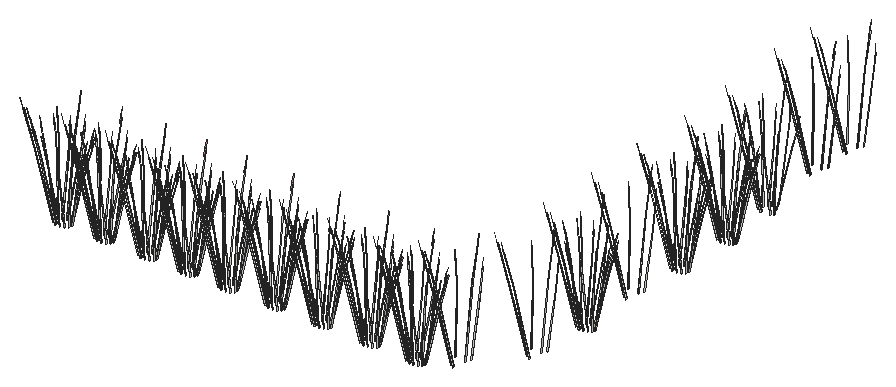
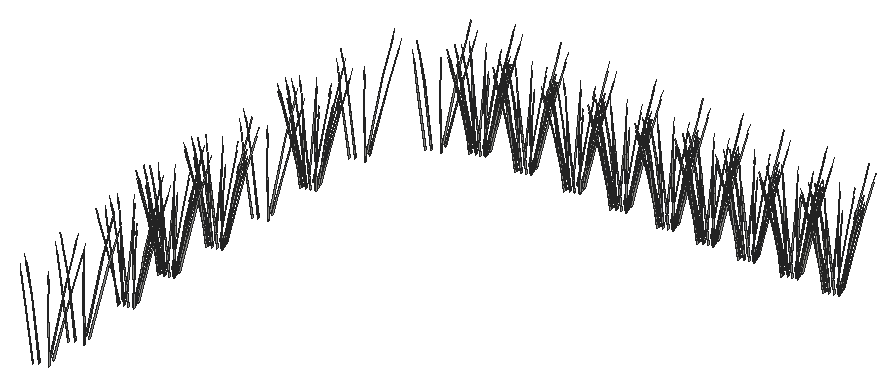
# SketchUp Ruby script. Lengths in inches.
U = 1.inch
M = Sketchup.active_model
def pt(a) = Geom::Point3d.new(a.map { |v| v * U })
def face(e, loops, mat)
  f = e.add_face(loops[0].map { |a| pt(a) })
  loops[1..].each { |l| e.add_face(l.map { |a| pt(a) }).erase! }
  f.material = f.back_material = mat if mat
  f
end
# faces: each face lists its corners as indices into pts; further lists are holes
def faces(e, pts, list, mat = nil) = list.each { |f| face(e, (f[0].is_a?(Array) ? f : [f]).map { |l| l.map { |i| pts[i] } }, mat) }
# xy, xz, yz: faces in a plane at the given z, y or x. An outline is a flat list of corners, or four numbers for a rectangle; further outlines are holes
def ring(l) = l.size == 4 ? [[l[0], l[1]], [l[2], l[1]], [l[2], l[3]], [l[0], l[3]]] : l.each_slice(2).to_a
def flat(e, list, mat, &to3) = list.each { |f| face(e, (f[0].is_a?(Array) ? f : [f]).map { |l| ring(l).map { |u, v| to3.(u, v) } }, mat) }
def xy(e, z, list, mat = nil) = flat(e, list, mat) { |x, y| [x, y, z] }
def xz(e, y, list, mat = nil) = flat(e, list, mat) { |x, z| [x, y, z] }
def yz(e, x, list, mat = nil) = flat(e, list, mat) { |y, z| [x, y, z] }
def lines(e, pts, list) = list.each { |a, b| e.add_line(pt(pts[a]), pt(pts[b])) }
# prism: a flat outline (further loops are holes) pulled along v
def prism(e, loops, v, mat = nil)
  f = face(e, loops, mat); d = Geom::Vector3d.new(v.map { |x| x * U })
  f.pushpull(f.normal.samedirection?(d) ? d.length : -d.length)
end
def box(e, o, s, mat = nil) = prism(e, [[o, [o[0] + s[0], o[1], o[2]], [o[0] + s[0], o[1] + s[1], o[2]], [o[0], o[1] + s[1], o[2]]]], [0, 0, s[2]], mat)
def at(x, y, z, deg = 0) = Geom::Transformation.translation(pt([x, y, z])) * Geom::Transformation.rotation(ORIGIN, Z_AXIS, deg.degrees)
def axes(o, x, y, z) = Geom::Transformation.new([*x, 0, *y, 0, *z, 0, *pt(o).to_a, 1])
def part(name) = M.definitions.add(name)
# library, detail: a bought-in or finely detailed component or shape, given as its bounding box
def library(name, o, s) = part(name).tap { |d| box(d.entities, o, s) }
def detail(e, o, s) = box(e.add_group.entities, o, s)
def put(e, d, t, mat = nil) = e.add_instance(d, t).tap { |i| i.material = mat if mat }
def group(e, t, mat = nil) = e.add_group.tap { |g| g.transformation = t; g.material = mat if mat }.entities
root = M.entities
M.materials.add("LightPink_Translucent").color = [144, 107, 117]
M.materials["LightPink_Translucent"].alpha = 0.75
c1 = part("blade")
p = [[2.15,0.21,22],[0,0.17,0],[0.09,0.45,0],[2.18,0.31,22],[2.29,0.31,22],[0.38,0.45,0],
  [2.48,0.24,33],[2.49,0.24,33],[2.48,0.22,33]]
faces(c1.entities,p,[[0,1,2,3],[4,5,2,3],[6,3,4,7],[8,0,3,6]])
c2 = part("seeds")
p = [[0.3,-0.1,1.38],[-0.01,-0.03,1.59],[-0.01,-0.03,0.03],[0.14,-0.07,-0.07],[0.29,-0.03,3],[0.15,0.01,3.11]]
faces(c2.entities,p,[[0,1,2,3],[1,0,4,5]],"LightPink_Translucent")
c3 = part("blade with seeds")
put(c3.entities,c1,at(0,0,0))
put(c3.entities,c2,axes([2.4,0.25,30.99],[1.5799,-0.05474,1.17369],[-0.12525,1.92788,0.29478],[-0.07173,-0.02425,1.56792]))
put(root,c3,axes([404.58,190.8125,260.05],[0.43232,0.38257,0.35414],[-0.49364,0.36215,-0.4572],[-0.25081,-0.0551,0.87481]))
put(root,c3,axes([404.87,194.07,260.05],[0.5141,-0.32171,0.35414],[0.48666,0.36734,-0.4572],[-0.07405,0.18664,0.87481]))
put(root,c3,axes([403.97,193.08,260.05],[0.66138,-0.08733,0.35414],[0.17464,0.49921,-0.4572],[-0.18953,0.13408,0.87481]))
put(root,c3,axes([407.91,194.52,260.05],[-0.11735,-0.49217,0.35414],[0.67083,-0.12996,-0.4572],[0.18018,0.14104,0.87481]))
put(root,c3,axes([409.85,191.59,260.05],[-0.66138,0.08733,0.35414],[-0.17464,-0.49921,-0.4572],[0.18953,-0.13408,0.87481]))
put(root,c3,axes([403.87,191.89,260.05],[0.63144,0.17046,0.35414],[-0.18417,0.49731,-0.4572],[-0.25423,0.0456,0.87481]))
put(root,c3,axes([408.96,190.6,260.05],[-0.5141,0.32171,0.35414],[-0.48666,-0.36734,-0.4572],[0.07405,-0.18664,0.87481]))
put(root,c3,axes([405.92,190.15,260.05],[0.11735,0.49217,0.35414],[-0.67083,0.12996,-0.4572],[-0.18018,-0.14104,0.87481]))
put(root,c3,axes([408.33,172.47,260.05],[0.22906,-0.4699,0.35414],[0.66828,0.13705,-0.4572],[0.06128,0.18919,0.87481]))
put(root,c3,axes([409.54,167.9375,260.05],[-0.22906,0.4699,0.35414],[-0.66828,-0.13705,-0.4572],[-0.06128,-0.18919,0.87481]))
put(root,c3,axes([411.27,171.73,260.05],[-0.43232,-0.38257,0.35414],[0.49364,-0.36215,-0.4572],[0.25081,0.0551,0.87481]))
put(root,c3,axes([411.98,170.66,260.05],[-0.63144,-0.17046,0.35414],[0.18417,-0.49731,-0.4572],[0.25423,-0.0456,0.87481]))
put(root,c3,axes([406.6,168.68,260.05],[0.43232,0.38257,0.35414],[-0.49364,0.36215,-0.4572],[-0.25081,-0.0551,0.87481]))
put(root,c3,axes([406.89,171.94,260.05],[0.5141,-0.32171,0.35414],[0.48666,0.36734,-0.4572],[-0.07405,0.18664,0.87481]))
put(root,c3,axes([405.99,170.95,260.05],[0.66138,-0.08733,0.35414],[0.17464,0.49921,-0.4572],[-0.18953,0.13408,0.87481]))
put(root,c3,axes([409.93,172.39,260.05],[-0.11735,-0.49217,0.35414],[0.67083,-0.12996,-0.4572],[0.18018,0.14104,0.87481]))
put(root,c3,axes([411.875,169.46,260.05],[-0.66138,0.08733,0.35414],[-0.17464,-0.49921,-0.4572],[0.18953,-0.13408,0.87481]))
put(root,c3,axes([405.89,169.75,260.05],[0.63144,0.17046,0.35414],[-0.18417,0.49731,-0.4572],[-0.25423,0.0456,0.87481]))
put(root,c3,axes([410.98,168.47,260.05],[-0.5141,0.32171,0.35414],[-0.48666,-0.36734,-0.4572],[0.07405,-0.18664,0.87481]))
put(root,c3,axes([407.93,168.02,260.05],[0.11735,0.49217,0.35414],[-0.67083,0.12996,-0.4572],[-0.18018,-0.14104,0.87481]))
put(root,c3,axes([407.96,149.88,260.05],[0.22906,-0.4699,0.35414],[0.66828,0.13705,-0.4572],[0.06128,0.18919,0.87481]))
put(root,c3,axes([409.18,145.35,260.05],[-0.22906,0.4699,0.35414],[-0.66828,-0.13705,-0.4572],[-0.06128,-0.18919,0.87481]))
put(root,c3,axes([410.91,149.14,260.05],[-0.43232,-0.38257,0.35414],[0.49364,-0.36215,-0.4572],[0.25081,0.0551,0.87481]))
put(root,c3,axes([411.62,148.0625,260.05],[-0.63144,-0.17046,0.35414],[0.18417,-0.49731,-0.4572],[0.25423,-0.0456,0.87481]))
put(root,c3,axes([406.24,146.09,260.05],[0.43232,0.38257,0.35414],[-0.49364,0.36215,-0.4572],[-0.25081,-0.0551,0.87481]))
put(root,c3,axes([406.52,149.35,260.05],[0.5141,-0.32171,0.35414],[0.48666,0.36734,-0.4572],[-0.07405,0.18664,0.87481]))
put(root,c3,axes([405.63,148.35,260.05],[0.66138,-0.08733,0.35414],[0.17464,0.49921,-0.4572],[-0.18953,0.13408,0.87481]))
put(root,c3,axes([409.57,149.8,260.05],[-0.11735,-0.49217,0.35414],[0.67083,-0.12996,-0.4572],[0.18018,0.14104,0.87481]))
put(root,c3,axes([411.51,146.87,260.05],[-0.66138,0.08733,0.35414],[-0.17464,-0.49921,-0.4572],[0.18953,-0.13408,0.87481]))
put(root,c3,axes([405.52,147.16,260.05],[0.63144,0.17046,0.35414],[-0.18417,0.49731,-0.4572],[-0.25423,0.0456,0.87481]))
put(root,c3,axes([410.62,145.875,260.05],[-0.5141,0.32171,0.35414],[-0.48666,-0.36734,-0.4572],[0.07405,-0.18664,0.87481]))
put(root,c3,axes([407.57,145.42,260.05],[0.11735,0.49217,0.35414],[-0.67083,0.12996,-0.4572],[-0.18018,-0.14104,0.87481]))
put(root,c3,axes([408.46,104.08,260.05],[0.22906,-0.4699,0.35414],[0.66828,0.13705,-0.4572],[0.06128,0.18919,0.87481]))
put(root,c3,axes([409.67,99.55,260.05],[-0.22906,0.4699,0.35414],[-0.66828,-0.13705,-0.4572],[-0.06128,-0.18919,0.87481]))
put(root,c3,axes([411.4,103.34,260.05],[-0.43232,-0.38257,0.35414],[0.49364,-0.36215,-0.4572],[0.25081,0.0551,0.87481]))
put(root,c3,axes([412.11,102.27,260.05],[-0.63144,-0.17046,0.35414],[0.18417,-0.49731,-0.4572],[0.25423,-0.0456,0.87481]))
put(root,c3,axes([406.73,100.29,260.05],[0.43232,0.38257,0.35414],[-0.49364,0.36215,-0.4572],[-0.25081,-0.0551,0.87481]))
put(root,c3,axes([407.02,103.55,260.05],[0.5141,-0.32171,0.35414],[0.48666,0.36734,-0.4572],[-0.07405,0.18664,0.87481]))
put(root,c3,axes([406.125,102.56,260.05],[0.66138,-0.08733,0.35414],[0.17464,0.49921,-0.4572],[-0.18953,0.13408,0.87481]))
put(root,c3,axes([410.07,104,260.05],[-0.11735,-0.49217,0.35414],[0.67083,-0.12996,-0.4572],[0.18018,0.14104,0.87481]))
put(root,c3,axes([412.01,101.07,260.05],[-0.66138,0.08733,0.35414],[-0.17464,-0.49921,-0.4572],[0.18953,-0.13408,0.87481]))
put(root,c3,axes([406.02,101.36,260.05],[0.63144,0.17046,0.35414],[-0.18417,0.49731,-0.4572],[-0.25423,0.0456,0.87481]))
put(root,c3,axes([411.12,100.08,260.05],[-0.5141,0.32171,0.35414],[-0.48666,-0.36734,-0.4572],[0.07405,-0.18664,0.87481]))
put(root,c3,axes([408.07,99.625,260.05],[0.11735,0.49217,0.35414],[-0.67083,0.12996,-0.4572],[-0.18018,-0.14104,0.87481]))
put(root,c3,axes([381.59,55.89,260.05],[0.22906,-0.4699,0.35414],[0.66828,0.13705,-0.4572],[0.06128,0.18919,0.87481]))
put(root,c3,axes([382.8,51.36,260.05],[-0.22906,0.4699,0.35414],[-0.66828,-0.13705,-0.4572],[-0.06128,-0.18919,0.87481]))
put(root,c3,axes([384.53,55.15,260.05],[-0.43232,-0.38257,0.35414],[0.49364,-0.36215,-0.4572],[0.25081,0.0551,0.87481]))
put(root,c3,axes([385.24,54.08,260.05],[-0.63144,-0.17046,0.35414],[0.18417,-0.49731,-0.4572],[0.25423,-0.0456,0.87481]))
put(root,c3,axes([379.86,52.1,260.05],[0.43232,0.38257,0.35414],[-0.49364,0.36215,-0.4572],[-0.25081,-0.0551,0.87481]))
put(root,c3,axes([380.15,55.37,260.05],[0.5141,-0.32171,0.35414],[0.48666,0.36734,-0.4572],[-0.07405,0.18664,0.87481]))
put(root,c3,axes([379.25,54.37,260.05],[0.66138,-0.08733,0.35414],[0.17464,0.49921,-0.4572],[-0.18953,0.13408,0.87481]))
put(root,c3,axes([383.19,55.82,260.05],[-0.11735,-0.49217,0.35414],[0.67083,-0.12996,-0.4572],[0.18018,0.14104,0.87481]))
put(root,c3,axes([385.14,52.89,260.05],[-0.66138,0.08733,0.35414],[-0.17464,-0.49921,-0.4572],[0.18953,-0.13408,0.87481]))
put(root,c3,axes([379.15,53.18,260.05],[0.63144,0.17046,0.35414],[-0.18417,0.49731,-0.4572],[-0.25423,0.0456,0.87481]))
put(root,c3,axes([384.24,51.89,260.05],[-0.5141,0.32171,0.35414],[-0.48666,-0.36734,-0.4572],[0.07405,-0.18664,0.87481]))
put(root,c3,axes([381.2,51.4375,260.05],[0.11735,0.49217,0.35414],[-0.67083,0.12996,-0.4572],[-0.18018,-0.14104,0.87481]))
put(root,c3,axes([363.95,55.89,260.05],[0.22906,-0.4699,0.35414],[0.66828,0.13705,-0.4572],[0.06128,0.18919,0.87481]))
put(root,c3,axes([365.16,51.36,260.05],[-0.22906,0.4699,0.35414],[-0.66828,-0.13705,-0.4572],[-0.06128,-0.18919,0.87481]))
put(root,c3,axes([366.89,55.15,260.05],[-0.43232,-0.38257,0.35414],[0.49364,-0.36215,-0.4572],[0.25081,0.0551,0.87481]))
put(root,c3,axes([367.6,54.08,260.05],[-0.63144,-0.17046,0.35414],[0.18417,-0.49731,-0.4572],[0.25423,-0.0456,0.87481]))
put(root,c3,axes([362.22,52.1,260.05],[0.43232,0.38257,0.35414],[-0.49364,0.36215,-0.4572],[-0.25081,-0.0551,0.87481]))
put(root,c3,axes([362.51,55.37,260.05],[0.5141,-0.32171,0.35414],[0.48666,0.36734,-0.4572],[-0.07405,0.18664,0.87481]))
put(root,c3,axes([361.62,54.37,260.05],[0.66138,-0.08733,0.35414],[0.17464,0.49921,-0.4572],[-0.18953,0.13408,0.87481]))
put(root,c3,axes([365.56,55.82,260.05],[-0.11735,-0.49217,0.35414],[0.67083,-0.12996,-0.4572],[0.18018,0.14104,0.87481]))
put(root,c3,axes([367.5,52.89,260.05],[-0.66138,0.08733,0.35414],[-0.17464,-0.49921,-0.4572],[0.18953,-0.13408,0.87481]))
put(root,c3,axes([361.51,53.18,260.05],[0.63144,0.17046,0.35414],[-0.18417,0.49731,-0.4572],[-0.25423,0.0456,0.87481]))
put(root,c3,axes([366.61,51.89,260.05],[-0.5141,0.32171,0.35414],[-0.48666,-0.36734,-0.4572],[0.07405,-0.18664,0.87481]))
put(root,c3,axes([363.5625,51.4375,260.05],[0.11735,0.49217,0.35414],[-0.67083,0.12996,-0.4572],[-0.18018,-0.14104,0.87481]))
put(root,c3,axes([345.17,55.89,260.05],[0.22906,-0.4699,0.35414],[0.66828,0.13705,-0.4572],[0.06128,0.18919,0.87481]))
put(root,c3,axes([346.38,51.36,260.05],[-0.22906,0.4699,0.35414],[-0.66828,-0.13705,-0.4572],[-0.06128,-0.18919,0.87481]))
put(root,c3,axes([348.11,55.15,260.05],[-0.43232,-0.38257,0.35414],[0.49364,-0.36215,-0.4572],[0.25081,0.0551,0.87481]))
put(root,c3,axes([348.82,54.08,260.05],[-0.63144,-0.17046,0.35414],[0.18417,-0.49731,-0.4572],[0.25423,-0.0456,0.87481]))
put(root,c3,axes([343.44,52.1,260.05],[0.43232,0.38257,0.35414],[-0.49364,0.36215,-0.4572],[-0.25081,-0.0551,0.87481]))
put(root,c3,axes([343.73,55.37,260.05],[0.5141,-0.32171,0.35414],[0.48666,0.36734,-0.4572],[-0.07405,0.18664,0.87481]))
put(root,c3,axes([342.84,54.37,260.05],[0.66138,-0.08733,0.35414],[0.17464,0.49921,-0.4572],[-0.18953,0.13408,0.87481]))
put(root,c3,axes([346.77,55.82,260.05],[-0.11735,-0.49217,0.35414],[0.67083,-0.12996,-0.4572],[0.18018,0.14104,0.87481]))
put(root,c3,axes([348.72,52.89,260.05],[-0.66138,0.08733,0.35414],[-0.17464,-0.49921,-0.4572],[0.18953,-0.13408,0.87481]))
put(root,c3,axes([342.73,53.18,260.05],[0.63144,0.17046,0.35414],[-0.18417,0.49731,-0.4572],[-0.25423,0.0456,0.87481]))
put(root,c3,axes([347.82,51.89,260.05],[-0.5141,0.32171,0.35414],[-0.48666,-0.36734,-0.4572],[0.07405,-0.18664,0.87481]))
put(root,c3,axes([344.78,51.4375,260.05],[0.11735,0.49217,0.35414],[-0.67083,0.12996,-0.4572],[-0.18018,-0.14104,0.87481]))
put(root,c3,axes([327.26,55.89,260.05],[0.22906,-0.4699,0.35414],[0.66828,0.13705,-0.4572],[0.06128,0.18919,0.87481]))
put(root,c3,axes([328.48,51.36,260.05],[-0.22906,0.4699,0.35414],[-0.66828,-0.13705,-0.4572],[-0.06128,-0.18919,0.87481]))
put(root,c3,axes([330.2,55.15,260.05],[-0.43232,-0.38257,0.35414],[0.49364,-0.36215,-0.4572],[0.25081,0.0551,0.87481]))
put(root,c3,axes([330.92,54.08,260.05],[-0.63144,-0.17046,0.35414],[0.18417,-0.49731,-0.4572],[0.25423,-0.0456,0.87481]))
put(root,c3,axes([325.54,52.1,260.05],[0.43232,0.38257,0.35414],[-0.49364,0.36215,-0.4572],[-0.25081,-0.0551,0.87481]))
put(root,c3,axes([325.82,55.37,260.05],[0.5141,-0.32171,0.35414],[0.48666,0.36734,-0.4572],[-0.07405,0.18664,0.87481]))
put(root,c3,axes([324.93,54.37,260.05],[0.66138,-0.08733,0.35414],[0.17464,0.49921,-0.4572],[-0.18953,0.13408,0.87481]))
put(root,c3,axes([328.87,55.82,260.05],[-0.11735,-0.49217,0.35414],[0.67083,-0.12996,-0.4572],[0.18018,0.14104,0.87481]))
put(root,c3,axes([330.8125,52.89,260.05],[-0.66138,0.08733,0.35414],[-0.17464,-0.49921,-0.4572],[0.18953,-0.13408,0.87481]))
put(root,c3,axes([324.82,53.18,260.05],[0.63144,0.17046,0.35414],[-0.18417,0.49731,-0.4572],[-0.25423,0.0456,0.87481]))
put(root,c3,axes([329.92,51.89,260.05],[-0.5141,0.32171,0.35414],[-0.48666,-0.36734,-0.4572],[0.07405,-0.18664,0.87481]))
put(root,c3,axes([326.87,51.4375,260.05],[0.11735,0.49217,0.35414],[-0.67083,0.12996,-0.4572],[-0.18018,-0.14104,0.87481]))
put(root,c3,axes([309.16,55.89,260.05],[0.22906,-0.4699,0.35414],[0.66828,0.13705,-0.4572],[0.06128,0.18919,0.87481]))
put(root,c3,axes([310.37,51.36,260.05],[-0.22906,0.4699,0.35414],[-0.66828,-0.13705,-0.4572],[-0.06128,-0.18919,0.87481]))
put(root,c3,axes([312.1,55.15,260.05],[-0.43232,-0.38257,0.35414],[0.49364,-0.36215,-0.4572],[0.25081,0.0551,0.87481]))
put(root,c3,axes([312.81,54.08,260.05],[-0.63144,-0.17046,0.35414],[0.18417,-0.49731,-0.4572],[0.25423,-0.0456,0.87481]))
put(root,c3,axes([307.43,52.1,260.05],[0.43232,0.38257,0.35414],[-0.49364,0.36215,-0.4572],[-0.25081,-0.0551,0.87481]))
put(root,c3,axes([307.71,55.37,260.05],[0.5141,-0.32171,0.35414],[0.48666,0.36734,-0.4572],[-0.07405,0.18664,0.87481]))
put(root,c3,axes([306.82,54.37,260.05],[0.66138,-0.08733,0.35414],[0.17464,0.49921,-0.4572],[-0.18953,0.13408,0.87481]))
put(root,c3,axes([310.76,55.82,260.05],[-0.11735,-0.49217,0.35414],[0.67083,-0.12996,-0.4572],[0.18018,0.14104,0.87481]))
put(root,c3,axes([312.7,52.89,260.05],[-0.66138,0.08733,0.35414],[-0.17464,-0.49921,-0.4572],[0.18953,-0.13408,0.87481]))
put(root,c3,axes([306.72,53.18,260.05],[0.63144,0.17046,0.35414],[-0.18417,0.49731,-0.4572],[-0.25423,0.0456,0.87481]))
put(root,c3,axes([311.81,51.89,260.05],[-0.5141,0.32171,0.35414],[-0.48666,-0.36734,-0.4572],[0.07405,-0.18664,0.87481]))
put(root,c3,axes([308.76,51.4375,260.05],[0.11735,0.49217,0.35414],[-0.67083,0.12996,-0.4572],[-0.18018,-0.14104,0.87481]))
put(root,c3,axes([293.71,55.89,260.05],[0.22906,-0.4699,0.35414],[0.66828,0.13705,-0.4572],[0.06128,0.18919,0.87481]))
put(root,c3,axes([294.92,51.36,260.05],[-0.22906,0.4699,0.35414],[-0.66828,-0.13705,-0.4572],[-0.06128,-0.18919,0.87481]))
put(root,c3,axes([296.65,55.15,260.05],[-0.43232,-0.38257,0.35414],[0.49364,-0.36215,-0.4572],[0.25081,0.0551,0.87481]))
put(root,c3,axes([297.36,54.08,260.05],[-0.63144,-0.17046,0.35414],[0.18417,-0.49731,-0.4572],[0.25423,-0.0456,0.87481]))
put(root,c3,axes([291.98,52.1,260.05],[0.43232,0.38257,0.35414],[-0.49364,0.36215,-0.4572],[-0.25081,-0.0551,0.87481]))
put(root,c3,axes([292.27,55.37,260.05],[0.5141,-0.32171,0.35414],[0.48666,0.36734,-0.4572],[-0.07405,0.18664,0.87481]))
put(root,c3,axes([291.375,54.37,260.05],[0.66138,-0.08733,0.35414],[0.17464,0.49921,-0.4572],[-0.18953,0.13408,0.87481]))
put(root,c3,axes([295.3125,55.82,260.05],[-0.11735,-0.49217,0.35414],[0.67083,-0.12996,-0.4572],[0.18018,0.14104,0.87481]))
put(root,c3,axes([297.25,52.89,260.05],[-0.66138,0.08733,0.35414],[-0.17464,-0.49921,-0.4572],[0.18953,-0.13408,0.87481]))
put(root,c3,axes([291.27,53.18,260.05],[0.63144,0.17046,0.35414],[-0.18417,0.49731,-0.4572],[-0.25423,0.0456,0.87481]))
put(root,c3,axes([296.36,51.89,260.05],[-0.5141,0.32171,0.35414],[-0.48666,-0.36734,-0.4572],[0.07405,-0.18664,0.87481]))
put(root,c3,axes([293.32,51.4375,260.05],[0.11735,0.49217,0.35414],[-0.67083,0.12996,-0.4572],[-0.18018,-0.14104,0.87481]))
put(root,c3,axes([277.98,55.89,260.05],[0.22906,-0.4699,0.35414],[0.66828,0.13705,-0.4572],[0.06128,0.18919,0.87481]))
put(root,c3,axes([279.19,51.36,260.05],[-0.22906,0.4699,0.35414],[-0.66828,-0.13705,-0.4572],[-0.06128,-0.18919,0.87481]))
put(root,c3,axes([280.92,55.15,260.05],[-0.43232,-0.38257,0.35414],[0.49364,-0.36215,-0.4572],[0.25081,0.0551,0.87481]))
put(root,c3,axes([281.63,54.08,260.05],[-0.63144,-0.17046,0.35414],[0.18417,-0.49731,-0.4572],[0.25423,-0.0456,0.87481]))
put(root,c3,axes([276.25,52.1,260.05],[0.43232,0.38257,0.35414],[-0.49364,0.36215,-0.4572],[-0.25081,-0.0551,0.87481]))
put(root,c3,axes([276.54,55.37,260.05],[0.5141,-0.32171,0.35414],[0.48666,0.36734,-0.4572],[-0.07405,0.18664,0.87481]))
put(root,c3,axes([275.65,54.37,260.05],[0.66138,-0.08733,0.35414],[0.17464,0.49921,-0.4572],[-0.18953,0.13408,0.87481]))
put(root,c3,axes([279.58,55.82,260.05],[-0.11735,-0.49217,0.35414],[0.67083,-0.12996,-0.4572],[0.18018,0.14104,0.87481]))
put(root,c3,axes([281.53,52.89,260.05],[-0.66138,0.08733,0.35414],[-0.17464,-0.49921,-0.4572],[0.18953,-0.13408,0.87481]))
put(root,c3,axes([275.54,53.18,260.05],[0.63144,0.17046,0.35414],[-0.18417,0.49731,-0.4572],[-0.25423,0.0456,0.87481]))
put(root,c3,axes([280.63,51.89,260.05],[-0.5141,0.32171,0.35414],[-0.48666,-0.36734,-0.4572],[0.07405,-0.18664,0.87481]))
put(root,c3,axes([277.59,51.4375,260.05],[0.11735,0.49217,0.35414],[-0.67083,0.12996,-0.4572],[-0.18018,-0.14104,0.87481]))
put(root,c3,axes([261.25,55.89,260.05],[0.22906,-0.4699,0.35414],[0.66828,0.13705,-0.4572],[0.06128,0.18919,0.87481]))
put(root,c3,axes([262.46,51.36,260.05],[-0.22906,0.4699,0.35414],[-0.66828,-0.13705,-0.4572],[-0.06128,-0.18919,0.87481]))
put(root,c3,axes([264.19,55.15,260.05],[-0.43232,-0.38257,0.35414],[0.49364,-0.36215,-0.4572],[0.25081,0.0551,0.87481]))
put(root,c3,axes([264.9,54.08,260.05],[-0.63144,-0.17046,0.35414],[0.18417,-0.49731,-0.4572],[0.25423,-0.0456,0.87481]))
put(root,c3,axes([259.52,52.1,260.05],[0.43232,0.38257,0.35414],[-0.49364,0.36215,-0.4572],[-0.25081,-0.0551,0.87481]))
put(root,c3,axes([259.81,55.37,260.05],[0.5141,-0.32171,0.35414],[0.48666,0.36734,-0.4572],[-0.07405,0.18664,0.87481]))
put(root,c3,axes([258.92,54.37,260.05],[0.66138,-0.08733,0.35414],[0.17464,0.49921,-0.4572],[-0.18953,0.13408,0.87481]))
put(root,c3,axes([262.86,55.82,260.05],[-0.11735,-0.49217,0.35414],[0.67083,-0.12996,-0.4572],[0.18018,0.14104,0.87481]))
put(root,c3,axes([264.8,52.89,260.05],[-0.66138,0.08733,0.35414],[-0.17464,-0.49921,-0.4572],[0.18953,-0.13408,0.87481]))
put(root,c3,axes([258.8125,53.18,260.05],[0.63144,0.17046,0.35414],[-0.18417,0.49731,-0.4572],[-0.25423,0.0456,0.87481]))
put(root,c3,axes([263.91,51.89,260.05],[-0.5141,0.32171,0.35414],[-0.48666,-0.36734,-0.4572],[0.07405,-0.18664,0.87481]))
put(root,c3,axes([260.86,51.4375,260.05],[0.11735,0.49217,0.35414],[-0.67083,0.12996,-0.4572],[-0.18018,-0.14104,0.87481]))
put(root,c3,axes([245.1875,55.89,260.05],[0.22906,-0.4699,0.35414],[0.66828,0.13705,-0.4572],[0.06128,0.18919,0.87481]))
put(root,c3,axes([246.4,51.36,260.05],[-0.22906,0.4699,0.35414],[-0.66828,-0.13705,-0.4572],[-0.06128,-0.18919,0.87481]))
put(root,c3,axes([248.13,55.15,260.05],[-0.43232,-0.38257,0.35414],[0.49364,-0.36215,-0.4572],[0.25081,0.0551,0.87481]))
put(root,c3,axes([248.84,54.08,260.05],[-0.63144,-0.17046,0.35414],[0.18417,-0.49731,-0.4572],[0.25423,-0.0456,0.87481]))
put(root,c3,axes([243.46,52.1,260.05],[0.43232,0.38257,0.35414],[-0.49364,0.36215,-0.4572],[-0.25081,-0.0551,0.87481]))
put(root,c3,axes([243.74,55.37,260.05],[0.5141,-0.32171,0.35414],[0.48666,0.36734,-0.4572],[-0.07405,0.18664,0.87481]))
put(root,c3,axes([242.85,54.37,260.05],[0.66138,-0.08733,0.35414],[0.17464,0.49921,-0.4572],[-0.18953,0.13408,0.87481]))
put(root,c3,axes([246.79,55.82,260.05],[-0.11735,-0.49217,0.35414],[0.67083,-0.12996,-0.4572],[0.18018,0.14104,0.87481]))
put(root,c3,axes([248.73,52.89,260.05],[-0.66138,0.08733,0.35414],[-0.17464,-0.49921,-0.4572],[0.18953,-0.13408,0.87481]))
put(root,c3,axes([242.75,53.18,260.05],[0.63144,0.17046,0.35414],[-0.18417,0.49731,-0.4572],[-0.25423,0.0456,0.87481]))
put(root,c3,axes([247.84,51.89,260.05],[-0.5141,0.32171,0.35414],[-0.48666,-0.36734,-0.4572],[0.07405,-0.18664,0.87481]))
put(root,c3,axes([244.79,51.4375,260.05],[0.11735,0.49217,0.35414],[-0.67083,0.12996,-0.4572],[-0.18018,-0.14104,0.87481]))
put(root,c3,axes([403.9,221.74,260.0625],[-0.74868,-0.15974,0.53283],[0.25601,-0.52518,0.43934],[0.04499,0.20653,1.10256]))
put(root,c3,axes([408.23,127.85,260.0625],[-0.74868,-0.15974,0.53283],[0.25601,-0.52518,0.43934],[0.04499,0.20653,1.10256]))
put(root,c3,axes([408.33,80.94,260.0625],[-0.74868,-0.15974,0.53283],[0.25601,-0.52518,0.43934],[0.04499,0.20653,1.10256]))
put(root,c3,axes([393.71,62.51,260.0625],[-0.74868,-0.15974,0.53283],[0.25601,-0.52518,0.43934],[0.04499,0.20653,1.10256]))
put(root,c3,axes([404.05,238.8125,260.0625],[-0.74868,-0.15974,0.53283],[0.25601,-0.52518,0.43934],[0.04499,0.20653,1.10256]))
put(root,c3,axes([406.3,194.99,260.0625],[-0.74868,-0.15974,0.53283],[0.25601,-0.52518,0.43934],[0.04499,0.20653,1.10256]))
put(root,c3,axes([408.32,172.86,260.0625],[-0.74868,-0.15974,0.53283],[0.25601,-0.52518,0.43934],[0.04499,0.20653,1.10256]))
put(root,c3,axes([407.96,150.26,260.0625],[-0.74868,-0.15974,0.53283],[0.25601,-0.52518,0.43934],[0.04499,0.20653,1.10256]))
put(root,c3,axes([408.45,104.47,260.0625],[-0.74868,-0.15974,0.53283],[0.25601,-0.52518,0.43934],[0.04499,0.20653,1.10256]))
put(root,c3,axes([381.58,56.28,260.0625],[-0.74868,-0.15974,0.53283],[0.25601,-0.52518,0.43934],[0.04499,0.20653,1.10256]))
put(root,c3,axes([363.94,56.28,260.0625],[-0.74868,-0.15974,0.53283],[0.25601,-0.52518,0.43934],[0.04499,0.20653,1.10256]))
put(root,c3,axes([345.16,56.28,260.0625],[-0.74868,-0.15974,0.53283],[0.25601,-0.52518,0.43934],[0.04499,0.20653,1.10256]))
put(root,c3,axes([327.25,56.28,260.0625],[-0.74868,-0.15974,0.53283],[0.25601,-0.52518,0.43934],[0.04499,0.20653,1.10256]))
put(root,c3,axes([309.15,56.28,260.0625],[-0.74868,-0.15974,0.53283],[0.25601,-0.52518,0.43934],[0.04499,0.20653,1.10256]))
put(root,c3,axes([293.7,56.28,260.0625],[-0.74868,-0.15974,0.53283],[0.25601,-0.52518,0.43934],[0.04499,0.20653,1.10256]))
put(root,c3,axes([277.97,56.28,260.0625],[-0.74868,-0.15974,0.53283],[0.25601,-0.52518,0.43934],[0.04499,0.20653,1.10256]))
put(root,c3,axes([261.24,56.28,260.0625],[-0.74868,-0.15974,0.53283],[0.25601,-0.52518,0.43934],[0.04499,0.20653,1.10256]))
put(root,c3,axes([245.18,56.28,260.0625],[-0.74868,-0.15974,0.53283],[0.25601,-0.52518,0.43934],[0.04499,0.20653,1.10256]))
put(root,c3,axes([401.5,217.22,260.09],[0.62747,-0.45094,0.53763],[0.54116,0.47889,0.4433],[-0.29439,-0.08318,1.11249]))
put(root,c3,axes([403.21,216.32,260.09],[0.84639,-0.15705,0.53763],[0.14689,0.61608,0.4433],[-0.19906,-0.18157,1.11249]))
put(root,c3,axes([405.84,123.33,260.09],[0.62747,-0.45094,0.53763],[0.54116,0.47889,0.4433],[-0.29439,-0.08318,1.11249]))
put(root,c3,axes([407.55,122.43,260.09],[0.84639,-0.15705,0.53763],[0.14689,0.61608,0.4433],[-0.19906,-0.18157,1.11249]))
put(root,c3,axes([405.93,76.42,260.09],[0.62747,-0.45094,0.53763],[0.54116,0.47889,0.4433],[-0.29439,-0.08318,1.11249]))
put(root,c3,axes([407.64,75.52,260.09],[0.84639,-0.15705,0.53763],[0.14689,0.61608,0.4433],[-0.19906,-0.18157,1.11249]))
put(root,c3,axes([391.3125,57.99,260.09],[0.62747,-0.45094,0.53763],[0.54116,0.47889,0.4433],[-0.29439,-0.08318,1.11249]))
put(root,c3,axes([393.03,57.09,260.09],[0.84639,-0.15705,0.53763],[0.14689,0.61608,0.4433],[-0.19906,-0.18157,1.11249]))
put(root,c3,axes([401.66,234.29,260.09],[0.62747,-0.45094,0.53763],[0.54116,0.47889,0.4433],[-0.29439,-0.08318,1.11249]))
put(root,c3,axes([403.37,233.39,260.09],[0.84639,-0.15705,0.53763],[0.14689,0.61608,0.4433],[-0.19906,-0.18157,1.11249]))
put(root,c3,axes([403.9,190.47,260.09],[0.62747,-0.45094,0.53763],[0.54116,0.47889,0.4433],[-0.29439,-0.08318,1.11249]))
put(root,c3,axes([405.61,189.57,260.09],[0.84639,-0.15705,0.53763],[0.14689,0.61608,0.4433],[-0.19906,-0.18157,1.11249]))
put(root,c3,axes([405.92,168.34,260.09],[0.62747,-0.45094,0.53763],[0.54116,0.47889,0.4433],[-0.29439,-0.08318,1.11249]))
put(root,c3,axes([407.63,167.4375,260.09],[0.84639,-0.15705,0.53763],[0.14689,0.61608,0.4433],[-0.19906,-0.18157,1.11249]))
put(root,c3,axes([405.56,145.74,260.09],[0.62747,-0.45094,0.53763],[0.54116,0.47889,0.4433],[-0.29439,-0.08318,1.11249]))
put(root,c3,axes([407.27,144.84,260.09],[0.84639,-0.15705,0.53763],[0.14689,0.61608,0.4433],[-0.19906,-0.18157,1.11249]))
put(root,c3,axes([406.05,99.95,260.09],[0.62747,-0.45094,0.53763],[0.54116,0.47889,0.4433],[-0.29439,-0.08318,1.11249]))
put(root,c3,axes([407.77,99.05,260.09],[0.84639,-0.15705,0.53763],[0.14689,0.61608,0.4433],[-0.19906,-0.18157,1.11249]))
put(root,c3,axes([379.18,51.76,260.09],[0.62747,-0.45094,0.53763],[0.54116,0.47889,0.4433],[-0.29439,-0.08318,1.11249]))
put(root,c3,axes([380.9,50.86,260.09],[0.84639,-0.15705,0.53763],[0.14689,0.61608,0.4433],[-0.19906,-0.18157,1.11249]))
put(root,c3,axes([361.55,51.76,260.09],[0.62747,-0.45094,0.53763],[0.54116,0.47889,0.4433],[-0.29439,-0.08318,1.11249]))
put(root,c3,axes([363.26,50.86,260.09],[0.84639,-0.15705,0.53763],[0.14689,0.61608,0.4433],[-0.19906,-0.18157,1.11249]))
put(root,c3,axes([342.76,51.76,260.09],[0.62747,-0.45094,0.53763],[0.54116,0.47889,0.4433],[-0.29439,-0.08318,1.11249]))
put(root,c3,axes([344.48,50.86,260.09],[0.84639,-0.15705,0.53763],[0.14689,0.61608,0.4433],[-0.19906,-0.18157,1.11249]))
put(root,c3,axes([324.86,51.76,260.09],[0.62747,-0.45094,0.53763],[0.54116,0.47889,0.4433],[-0.29439,-0.08318,1.11249]))
put(root,c3,axes([326.57,50.86,260.09],[0.84639,-0.15705,0.53763],[0.14689,0.61608,0.4433],[-0.19906,-0.18157,1.11249]))
put(root,c3,axes([306.75,51.76,260.09],[0.62747,-0.45094,0.53763],[0.54116,0.47889,0.4433],[-0.29439,-0.08318,1.11249]))
put(root,c3,axes([308.46,50.86,260.09],[0.84639,-0.15705,0.53763],[0.14689,0.61608,0.4433],[-0.19906,-0.18157,1.11249]))
put(root,c3,axes([291.3,51.76,260.09],[0.62747,-0.45094,0.53763],[0.54116,0.47889,0.4433],[-0.29439,-0.08318,1.11249]))
put(root,c3,axes([293.01,50.86,260.09],[0.84639,-0.15705,0.53763],[0.14689,0.61608,0.4433],[-0.19906,-0.18157,1.11249]))
put(root,c3,axes([275.57,51.76,260.09],[0.62747,-0.45094,0.53763],[0.54116,0.47889,0.4433],[-0.29439,-0.08318,1.11249]))
put(root,c3,axes([277.29,50.86,260.09],[0.84639,-0.15705,0.53763],[0.14689,0.61608,0.4433],[-0.19906,-0.18157,1.11249]))
put(root,c3,axes([258.85,51.76,260.09],[0.62747,-0.45094,0.53763],[0.54116,0.47889,0.4433],[-0.29439,-0.08318,1.11249]))
put(root,c3,axes([260.56,50.86,260.09],[0.84639,-0.15705,0.53763],[0.14689,0.61608,0.4433],[-0.19906,-0.18157,1.11249]))
put(root,c3,axes([242.78,51.76,260.09],[0.62747,-0.45094,0.53763],[0.54116,0.47889,0.4433],[-0.29439,-0.08318,1.11249]))
put(root,c3,axes([244.49,50.86,260.09],[0.84639,-0.15705,0.53763],[0.14689,0.61608,0.4433],[-0.19906,-0.18157,1.11249]))
put(root,c3,axes([404.8,223.03,260.65],[0.52505,-0.35054,-0.06488],[0.48109,0.38392,-0.29416],[0.03387,0.10878,0.97024]))
put(root,c3,axes([400.07,221.25,260.65],[0.67048,0.16311,-0.06488],[-0.20625,0.50201,-0.29416],[-0.10966,0.07622,0.97024]))
put(root,c3,axes([409.14,129.14,260.65],[0.52505,-0.35054,-0.06488],[0.48109,0.38392,-0.29416],[0.03387,0.10878,0.97024]))
put(root,c3,axes([404.41,127.36,260.65],[0.67048,0.16311,-0.06488],[-0.20625,0.50201,-0.29416],[-0.10966,0.07622,0.97024]))
put(root,c3,axes([409.24,82.23,260.65],[0.52505,-0.35054,-0.06488],[0.48109,0.38392,-0.29416],[0.03387,0.10878,0.97024]))
put(root,c3,axes([404.5,80.45,260.65],[0.67048,0.16311,-0.06488],[-0.20625,0.50201,-0.29416],[-0.10966,0.07622,0.97024]))
put(root,c3,axes([394.62,63.8,260.65],[0.52505,-0.35054,-0.06488],[0.48109,0.38392,-0.29416],[0.03387,0.10878,0.97024]))
put(root,c3,axes([389.88,62.02,260.65],[0.67048,0.16311,-0.06488],[-0.20625,0.50201,-0.29416],[-0.10966,0.07622,0.97024]))
put(root,c3,axes([404.96,240.1,260.65],[0.52505,-0.35054,-0.06488],[0.48109,0.38392,-0.29416],[0.03387,0.10878,0.97024]))
put(root,c3,axes([400.23,238.32,260.65],[0.67048,0.16311,-0.06488],[-0.20625,0.50201,-0.29416],[-0.10966,0.07622,0.97024]))
put(root,c3,axes([407.21,196.28,260.65],[0.52505,-0.35054,-0.06488],[0.48109,0.38392,-0.29416],[0.03387,0.10878,0.97024]))
put(root,c3,axes([402.47,194.5,260.65],[0.67048,0.16311,-0.06488],[-0.20625,0.50201,-0.29416],[-0.10966,0.07622,0.97024]))
put(root,c3,axes([409.23,174.15,260.65],[0.52505,-0.35054,-0.06488],[0.48109,0.38392,-0.29416],[0.03387,0.10878,0.97024]))
put(root,c3,axes([404.49,172.37,260.65],[0.67048,0.16311,-0.06488],[-0.20625,0.50201,-0.29416],[-0.10966,0.07622,0.97024]))
put(root,c3,axes([408.86,151.55,260.65],[0.52505,-0.35054,-0.06488],[0.48109,0.38392,-0.29416],[0.03387,0.10878,0.97024]))
put(root,c3,axes([404.13,149.77,260.65],[0.67048,0.16311,-0.06488],[-0.20625,0.50201,-0.29416],[-0.10966,0.07622,0.97024]))
put(root,c3,axes([409.36,105.76,260.65],[0.52505,-0.35054,-0.06488],[0.48109,0.38392,-0.29416],[0.03387,0.10878,0.97024]))
put(root,c3,axes([404.625,103.98,260.65],[0.67048,0.16311,-0.06488],[-0.20625,0.50201,-0.29416],[-0.10966,0.07622,0.97024]))
put(root,c3,axes([382.49,57.57,260.65],[0.52505,-0.35054,-0.06488],[0.48109,0.38392,-0.29416],[0.03387,0.10878,0.97024]))
put(root,c3,axes([377.75,55.79,260.65],[0.67048,0.16311,-0.06488],[-0.20625,0.50201,-0.29416],[-0.10966,0.07622,0.97024]))
put(root,c3,axes([364.85,57.57,260.65],[0.52505,-0.35054,-0.06488],[0.48109,0.38392,-0.29416],[0.03387,0.10878,0.97024]))
put(root,c3,axes([360.12,55.79,260.65],[0.67048,0.16311,-0.06488],[-0.20625,0.50201,-0.29416],[-0.10966,0.07622,0.97024]))
put(root,c3,axes([346.07,57.57,260.65],[0.52505,-0.35054,-0.06488],[0.48109,0.38392,-0.29416],[0.03387,0.10878,0.97024]))
put(root,c3,axes([341.33,55.79,260.65],[0.67048,0.16311,-0.06488],[-0.20625,0.50201,-0.29416],[-0.10966,0.07622,0.97024]))
put(root,c3,axes([328.16,57.57,260.65],[0.52505,-0.35054,-0.06488],[0.48109,0.38392,-0.29416],[0.03387,0.10878,0.97024]))
put(root,c3,axes([323.43,55.79,260.65],[0.67048,0.16311,-0.06488],[-0.20625,0.50201,-0.29416],[-0.10966,0.07622,0.97024]))
put(root,c3,axes([310.06,57.57,260.65],[0.52505,-0.35054,-0.06488],[0.48109,0.38392,-0.29416],[0.03387,0.10878,0.97024]))
put(root,c3,axes([305.32,55.79,260.65],[0.67048,0.16311,-0.06488],[-0.20625,0.50201,-0.29416],[-0.10966,0.07622,0.97024]))
put(root,c3,axes([294.61,57.57,260.65],[0.52505,-0.35054,-0.06488],[0.48109,0.38392,-0.29416],[0.03387,0.10878,0.97024]))
put(root,c3,axes([289.87,55.79,260.65],[0.67048,0.16311,-0.06488],[-0.20625,0.50201,-0.29416],[-0.10966,0.07622,0.97024]))
put(root,c3,axes([278.88,57.57,260.65],[0.52505,-0.35054,-0.06488],[0.48109,0.38392,-0.29416],[0.03387,0.10878,0.97024]))
put(root,c3,axes([274.14,55.79,260.65],[0.67048,0.16311,-0.06488],[-0.20625,0.50201,-0.29416],[-0.10966,0.07622,0.97024]))
put(root,c3,axes([262.15,57.57,260.65],[0.52505,-0.35054,-0.06488],[0.48109,0.38392,-0.29416],[0.03387,0.10878,0.97024]))
put(root,c3,axes([257.42,55.79,260.65],[0.67048,0.16311,-0.06488],[-0.20625,0.50201,-0.29416],[-0.10966,0.07622,0.97024]))
put(root,c3,axes([246.09,57.57,260.65],[0.52505,-0.35054,-0.06488],[0.48109,0.38392,-0.29416],[0.03387,0.10878,0.97024]))
put(root,c3,axes([241.35,55.79,260.65],[0.67048,0.16311,-0.06488],[-0.20625,0.50201,-0.29416],[-0.10966,0.07622,0.97024]))
